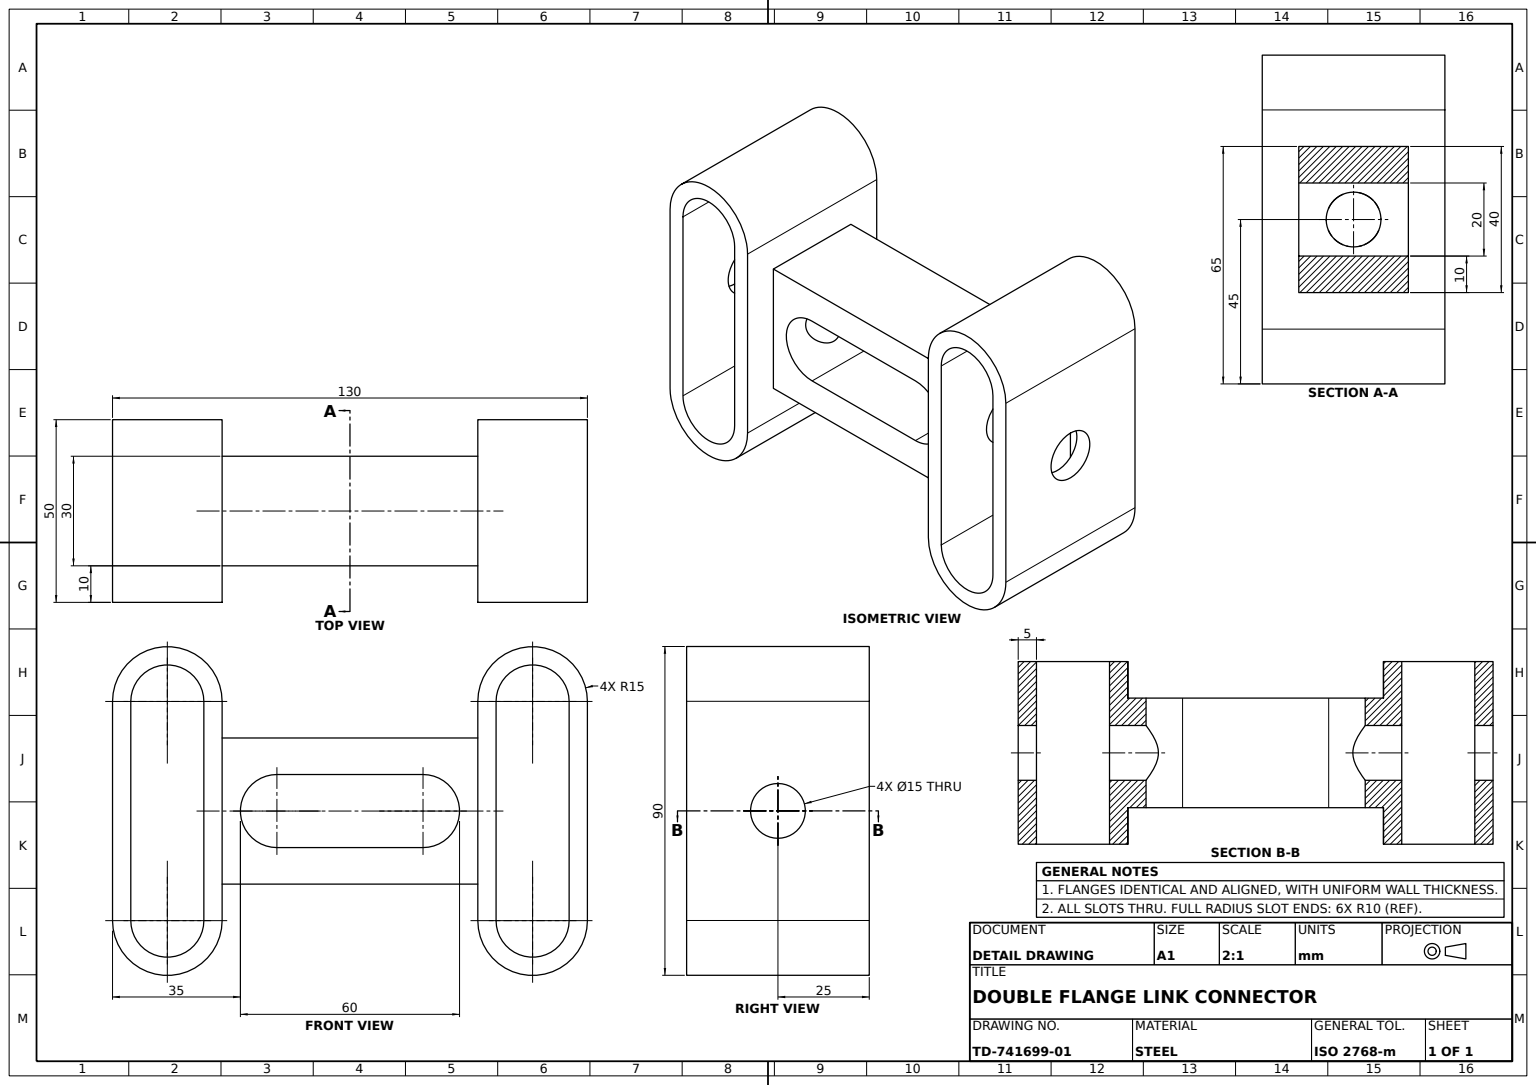
ISO-10303-21;
HEADER;
FILE_DESCRIPTION((''),'2;1');
FILE_NAME('','',(''),(''),'','','');
FILE_SCHEMA(('AUTOMOTIVE_DESIGN'));
ENDSEC;
DATA;
#1=APPLICATION_CONTEXT('');
#2=PRODUCT_CONTEXT('',#1,'mechanical');
#3=PRODUCT('','','',(#2));
#4=PRODUCT_DEFINITION_FORMATION('','',#3);
#5=PRODUCT_DEFINITION_CONTEXT('',#1,'design');
#6=PRODUCT_DEFINITION('','',#4,#5);
#7=PRODUCT_DEFINITION_SHAPE('','',#6);
#8=(LENGTH_UNIT()NAMED_UNIT(*)SI_UNIT(.MILLI.,.METRE.));
#9=(NAMED_UNIT(*)PLANE_ANGLE_UNIT()SI_UNIT($,.RADIAN.));
#10=(NAMED_UNIT(*)SI_UNIT($,.STERADIAN.)SOLID_ANGLE_UNIT());
#11=UNCERTAINTY_MEASURE_WITH_UNIT(LENGTH_MEASURE(0.005),#8,'distance_accuracy_value','');
#12=(GEOMETRIC_REPRESENTATION_CONTEXT(3)GLOBAL_UNCERTAINTY_ASSIGNED_CONTEXT((#11))GLOBAL_UNIT_ASSIGNED_CONTEXT((#8,#9,#10))REPRESENTATION_CONTEXT('',''));
#13=CARTESIAN_POINT('',(35.,15.,-20.));
#14=VERTEX_POINT('',#13);
#15=CARTESIAN_POINT('',(-35.,15.,-20.));
#16=VERTEX_POINT('',#15);
#17=CARTESIAN_POINT('',(65.,15.,-20.));
#18=DIRECTION('',(-1.,0.,0.));
#19=VECTOR('',#18,1000.);
#20=LINE('',#17,#19);
#21=EDGE_CURVE('',#14,#16,#20,.T.);
#22=ORIENTED_EDGE('',*,*,#21,.F.);
#23=CARTESIAN_POINT('',(35.,-15.,-20.));
#24=VERTEX_POINT('',#23);
#25=DIRECTION('',(0.,-1.,0.));
#26=VECTOR('',#25,1000.);
#27=LINE('',#23,#26);
#28=EDGE_CURVE('',#14,#24,#27,.T.);
#29=ORIENTED_EDGE('',*,*,#28,.T.);
#30=CARTESIAN_POINT('',(-35.,-15.,-20.));
#31=VERTEX_POINT('',#30);
#32=CARTESIAN_POINT('',(65.,-15.,-20.));
#33=LINE('',#32,#19);
#34=EDGE_CURVE('',#24,#31,#33,.T.);
#35=ORIENTED_EDGE('',*,*,#34,.T.);
#36=LINE('',#30,#26);
#37=EDGE_CURVE('',#16,#31,#36,.T.);
#38=ORIENTED_EDGE('',*,*,#37,.F.);
#39=EDGE_LOOP('',(#22,#29,#35,#38));
#40=FACE_BOUND('',#39,.T.);
#41=DIRECTION('',(0.,0.,-1.));
#42=AXIS2_PLACEMENT_3D('',#32,#41,#18);
#43=PLANE('',#42);
#44=ADVANCED_FACE('',(#40),#43,.T.);
#45=CARTESIAN_POINT('',(60.,25.,-30.));
#46=VERTEX_POINT('',#45);
#47=CARTESIAN_POINT('',(60.,-25.,-30.));
#48=VERTEX_POINT('',#47);
#49=CARTESIAN_POINT('',(60.,-51.,-30.));
#50=DIRECTION('',(0.,1.,0.));
#51=VECTOR('',#50,1000.);
#52=LINE('',#49,#51);
#53=EDGE_CURVE('',#46,#48,#52,.F.);
#54=ORIENTED_EDGE('',*,*,#53,.T.);
#55=CARTESIAN_POINT('',(60.,-25.,30.));
#56=VERTEX_POINT('',#55);
#57=VECTOR('',#41,1000.);
#58=LINE('',#55,#57);
#59=EDGE_CURVE('',#56,#48,#58,.T.);
#60=ORIENTED_EDGE('',*,*,#59,.F.);
#61=CARTESIAN_POINT('',(60.,25.,30.));
#62=VERTEX_POINT('',#61);
#63=CARTESIAN_POINT('',(60.,-51.,30.));
#64=LINE('',#63,#51);
#65=EDGE_CURVE('',#62,#56,#64,.F.);
#66=ORIENTED_EDGE('',*,*,#65,.F.);
#67=LINE('',#61,#57);
#68=EDGE_CURVE('',#62,#46,#67,.T.);
#69=ORIENTED_EDGE('',*,*,#68,.T.);
#70=EDGE_LOOP('',(#54,#60,#66,#69));
#71=FACE_BOUND('',#70,.T.);
#72=CARTESIAN_POINT('',(60.,0.,7.5));
#73=VERTEX_POINT('',#72);
#74=CARTESIAN_POINT('',(60.,0.,0.));
#75=DIRECTION('',(0.,0.,1.));
#76=AXIS2_PLACEMENT_3D('',#74,#18,#75);
#77=CIRCLE('',#76,7.5);
#78=EDGE_CURVE('',#73,#73,#77,.T.);
#79=ORIENTED_EDGE('',*,*,#78,.F.);
#80=EDGE_LOOP('',(#79));
#81=FACE_BOUND('',#80,.T.);
#82=AXIS2_PLACEMENT_3D('',#49,#18,#75);
#83=PLANE('',#82);
#84=ADVANCED_FACE('',(#71,#81),#83,.T.);
#85=CARTESIAN_POINT('',(40.,25.,-30.));
#86=VERTEX_POINT('',#85);
#87=CARTESIAN_POINT('',(50.,25.,-30.));
#88=AXIS2_PLACEMENT_3D('',#87,#25,#41);
#89=CIRCLE('',#88,10.);
#90=EDGE_CURVE('',#46,#86,#89,.F.);
#91=ORIENTED_EDGE('',*,*,#90,.T.);
#92=CARTESIAN_POINT('',(40.,-25.,-30.));
#93=VERTEX_POINT('',#92);
#94=CARTESIAN_POINT('',(40.,-51.,-30.));
#95=LINE('',#94,#51);
#96=EDGE_CURVE('',#86,#93,#95,.F.);
#97=ORIENTED_EDGE('',*,*,#96,.T.);
#98=CARTESIAN_POINT('',(50.,-25.,-30.));
#99=AXIS2_PLACEMENT_3D('',#98,#25,#41);
#100=CIRCLE('',#99,10.);
#101=EDGE_CURVE('',#48,#93,#100,.F.);
#102=ORIENTED_EDGE('',*,*,#101,.F.);
#103=ORIENTED_EDGE('',*,*,#53,.F.);
#104=EDGE_LOOP('',(#91,#97,#102,#103));
#105=FACE_BOUND('',#104,.T.);
#106=CARTESIAN_POINT('',(50.,-51.,-30.));
#107=AXIS2_PLACEMENT_3D('',#106,#50,#75);
#108=CYLINDRICAL_SURFACE('',#107,10.);
#109=ADVANCED_FACE('',(#105),#108,.F.);
#110=CARTESIAN_POINT('',(40.,0.,-7.5));
#111=VERTEX_POINT('',#110);
#112=CARTESIAN_POINT('',(40.,0.,0.));
#113=DIRECTION('',(1.,0.,0.));
#114=AXIS2_PLACEMENT_3D('',#112,#113,#41);
#115=CIRCLE('',#114,7.5);
#116=EDGE_CURVE('',#111,#111,#115,.T.);
#117=ORIENTED_EDGE('',*,*,#116,.T.);
#118=EDGE_LOOP('',(#117));
#119=FACE_BOUND('',#118,.T.);
#120=CARTESIAN_POINT('',(26.614378,0.,7.5));
#121=VERTEX_POINT('',#120);
#122=CARTESIAN_POINT('',(26.742202,-1.555656,7.390074));
#123=CARTESIAN_POINT('',(26.485198,0.527121,7.609599));
#124=CARTESIAN_POINT('',(27.137881,3.034196,7.063234));
#125=CARTESIAN_POINT('',(28.483267,5.377309,5.469181));
#126=CARTESIAN_POINT('',(29.650344,7.042163,3.112347));
#127=CARTESIAN_POINT('',(30.169282,7.721606,0.025455));
#128=CARTESIAN_POINT('',(29.672301,7.07111,-3.048672));
#129=CARTESIAN_POINT('',(28.494965,5.399488,-5.454098));
#130=CARTESIAN_POINT('',(27.380453,3.448516,-6.78143));
#131=CARTESIAN_POINT('',(26.74576,1.568514,-7.386559));
#132=CARTESIAN_POINT('',(26.551514,0.025291,-7.554237));
#133=CARTESIAN_POINT('',(26.734722,-1.523498,-7.396257));
#134=CARTESIAN_POINT('',(27.362431,-3.412182,-6.800946));
#135=CARTESIAN_POINT('',(28.477733,-5.372733,-5.475881));
#136=CARTESIAN_POINT('',(29.649907,-7.040721,-3.116164));
#137=CARTESIAN_POINT('',(30.169729,-7.722462,-0.025289));
#138=CARTESIAN_POINT('',(29.670957,-7.069137,3.05425));
#139=CARTESIAN_POINT('',(28.490958,-5.394144,5.460679));
#140=CARTESIAN_POINT('',(27.374214,-3.434962,6.787838));
#141=B_SPLINE_CURVE_WITH_KNOTS('',3,(#122,#123,#124,#125,#126,#127,#128,#129,#130,#131,#132,#133,#134,#135,#136,#137,#138,#139,#140,#122,#123,#124),.UNSPECIFIED.,.T.,.F.,(1,1,1,1,1,1,1,1,1,1,1,1,1,1,1,1,1,1,1,1,1,1,1,1,1,1),(-0.006118289,-0.003059145,-0.001529572,0.,0.003059145,0.006118289,0.009177434,0.012236578,0.015295723,0.018354867,0.021414012,0.022943584,0.024473156,0.026002728,0.027532301,0.030591445,0.03365059,0.036709734,0.039768879,0.042828023,0.045887168,0.04741674,0.048946312,0.052005457,0.055064601,0.058123746),.UNSPECIFIED.);
#142=EDGE_CURVE('',#121,#121,#141,.T.);
#143=ORIENTED_EDGE('',*,*,#142,.T.);
#144=EDGE_LOOP('',(#143));
#145=FACE_BOUND('',#144,.T.);
#146=CARTESIAN_POINT('',(65.,0.,0.));
#147=AXIS2_PLACEMENT_3D('',#146,#18,#75);
#148=CYLINDRICAL_SURFACE('',#147,7.5);
#149=ADVANCED_FACE('',(#119,#145),#148,.F.);
#150=ORIENTED_EDGE('',*,*,#78,.T.);
#151=EDGE_LOOP('',(#150));
#152=FACE_BOUND('',#151,.T.);
#153=CARTESIAN_POINT('',(65.,0.,7.5));
#154=VERTEX_POINT('',#153);
#155=CIRCLE('',#147,7.5);
#156=EDGE_CURVE('',#154,#154,#155,.T.);
#157=ORIENTED_EDGE('',*,*,#156,.F.);
#158=EDGE_LOOP('',(#157));
#159=FACE_BOUND('',#158,.T.);
#160=ADVANCED_FACE('',(#152,#159),#148,.F.);
#161=CARTESIAN_POINT('',(20.,15.,10.));
#162=VERTEX_POINT('',#161);
#163=CARTESIAN_POINT('',(20.,-15.,10.));
#164=VERTEX_POINT('',#163);
#165=CARTESIAN_POINT('',(20.,-51.,10.));
#166=LINE('',#165,#51);
#167=EDGE_CURVE('',#162,#164,#166,.F.);
#168=ORIENTED_EDGE('',*,*,#167,.T.);
#169=CARTESIAN_POINT('',(-20.,-15.,10.));
#170=VERTEX_POINT('',#169);
#171=CARTESIAN_POINT('',(0.,-15.,10.));
#172=LINE('',#171,#19);
#173=EDGE_CURVE('',#164,#170,#172,.T.);
#174=ORIENTED_EDGE('',*,*,#173,.T.);
#175=CARTESIAN_POINT('',(-20.,15.,10.));
#176=VERTEX_POINT('',#175);
#177=CARTESIAN_POINT('',(-20.,-51.,10.));
#178=LINE('',#177,#51);
#179=EDGE_CURVE('',#176,#170,#178,.F.);
#180=ORIENTED_EDGE('',*,*,#179,.F.);
#181=CARTESIAN_POINT('',(0.,15.,10.));
#182=LINE('',#181,#19);
#183=EDGE_CURVE('',#162,#176,#182,.T.);
#184=ORIENTED_EDGE('',*,*,#183,.F.);
#185=EDGE_LOOP('',(#168,#174,#180,#184));
#186=FACE_BOUND('',#185,.T.);
#187=AXIS2_PLACEMENT_3D('',#165,#41,#18);
#188=PLANE('',#187);
#189=ADVANCED_FACE('',(#186),#188,.T.);
#190=CARTESIAN_POINT('',(65.,25.,30.));
#191=VERTEX_POINT('',#190);
#192=CARTESIAN_POINT('',(35.,25.,30.));
#193=VERTEX_POINT('',#192);
#194=CARTESIAN_POINT('',(50.,25.,30.));
#195=AXIS2_PLACEMENT_3D('',#194,#25,#113);
#196=CIRCLE('',#195,15.);
#197=EDGE_CURVE('',#191,#193,#196,.T.);
#198=ORIENTED_EDGE('',*,*,#197,.F.);
#199=CARTESIAN_POINT('',(65.,25.,-30.));
#200=VERTEX_POINT('',#199);
#201=VECTOR('',#75,1000.);
#202=LINE('',#199,#201);
#203=EDGE_CURVE('',#200,#191,#202,.T.);
#204=ORIENTED_EDGE('',*,*,#203,.F.);
#205=CARTESIAN_POINT('',(35.,25.,-30.));
#206=VERTEX_POINT('',#205);
#207=AXIS2_PLACEMENT_3D('',#87,#25,#113);
#208=CIRCLE('',#207,15.);
#209=EDGE_CURVE('',#206,#200,#208,.T.);
#210=ORIENTED_EDGE('',*,*,#209,.F.);
#211=LINE('',#192,#57);
#212=EDGE_CURVE('',#193,#206,#211,.T.);
#213=ORIENTED_EDGE('',*,*,#212,.F.);
#214=EDGE_LOOP('',(#198,#204,#210,#213));
#215=FACE_BOUND('',#214,.T.);
#216=CARTESIAN_POINT('',(40.,25.,30.));
#217=VERTEX_POINT('',#216);
#218=AXIS2_PLACEMENT_3D('',#194,#25,#41);
#219=CIRCLE('',#218,10.);
#220=EDGE_CURVE('',#217,#62,#219,.F.);
#221=ORIENTED_EDGE('',*,*,#220,.F.);
#222=LINE('',#216,#201);
#223=EDGE_CURVE('',#86,#217,#222,.T.);
#224=ORIENTED_EDGE('',*,*,#223,.F.);
#225=ORIENTED_EDGE('',*,*,#90,.F.);
#226=ORIENTED_EDGE('',*,*,#68,.F.);
#227=EDGE_LOOP('',(#221,#224,#225,#226));
#228=FACE_BOUND('',#227,.T.);
#229=PLANE('',#218);
#230=ADVANCED_FACE('',(#215,#228),#229,.F.);
#231=CARTESIAN_POINT('',(-60.,0.,7.5));
#232=VERTEX_POINT('',#231);
#233=CARTESIAN_POINT('',(-60.,0.,0.));
#234=AXIS2_PLACEMENT_3D('',#233,#18,#75);
#235=CIRCLE('',#234,7.5);
#236=EDGE_CURVE('',#232,#232,#235,.T.);
#237=ORIENTED_EDGE('',*,*,#236,.T.);
#238=EDGE_LOOP('',(#237));
#239=FACE_BOUND('',#238,.T.);
#240=CARTESIAN_POINT('',(-60.,-25.,-30.));
#241=VERTEX_POINT('',#240);
#242=CARTESIAN_POINT('',(-60.,-25.,30.));
#243=VERTEX_POINT('',#242);
#244=LINE('',#242,#201);
#245=EDGE_CURVE('',#241,#243,#244,.T.);
#246=ORIENTED_EDGE('',*,*,#245,.F.);
#247=CARTESIAN_POINT('',(-60.,25.,-30.));
#248=VERTEX_POINT('',#247);
#249=CARTESIAN_POINT('',(-60.,-51.,-30.));
#250=LINE('',#249,#51);
#251=EDGE_CURVE('',#248,#241,#250,.F.);
#252=ORIENTED_EDGE('',*,*,#251,.F.);
#253=CARTESIAN_POINT('',(-60.,25.,30.));
#254=VERTEX_POINT('',#253);
#255=LINE('',#253,#201);
#256=EDGE_CURVE('',#248,#254,#255,.T.);
#257=ORIENTED_EDGE('',*,*,#256,.T.);
#258=CARTESIAN_POINT('',(-60.,-51.,30.));
#259=LINE('',#258,#51);
#260=EDGE_CURVE('',#254,#243,#259,.F.);
#261=ORIENTED_EDGE('',*,*,#260,.T.);
#262=EDGE_LOOP('',(#246,#252,#257,#261));
#263=FACE_BOUND('',#262,.T.);
#264=AXIS2_PLACEMENT_3D('',#249,#18,#75);
#265=PLANE('',#264);
#266=ADVANCED_FACE('',(#239,#263),#265,.F.);
#267=ORIENTED_EDGE('',*,*,#220,.T.);
#268=ORIENTED_EDGE('',*,*,#65,.T.);
#269=CARTESIAN_POINT('',(40.,-25.,30.));
#270=VERTEX_POINT('',#269);
#271=CARTESIAN_POINT('',(50.,-25.,30.));
#272=AXIS2_PLACEMENT_3D('',#271,#25,#41);
#273=CIRCLE('',#272,10.);
#274=EDGE_CURVE('',#270,#56,#273,.F.);
#275=ORIENTED_EDGE('',*,*,#274,.F.);
#276=CARTESIAN_POINT('',(40.,-51.,30.));
#277=LINE('',#276,#51);
#278=EDGE_CURVE('',#217,#270,#277,.F.);
#279=ORIENTED_EDGE('',*,*,#278,.F.);
#280=EDGE_LOOP('',(#267,#268,#275,#279));
#281=FACE_BOUND('',#280,.T.);
#282=CARTESIAN_POINT('',(50.,-51.,30.));
#283=AXIS2_PLACEMENT_3D('',#282,#50,#75);
#284=CYLINDRICAL_SURFACE('',#283,10.);
#285=ADVANCED_FACE('',(#281),#284,.F.);
#286=ORIENTED_EDGE('',*,*,#116,.F.);
#287=EDGE_LOOP('',(#286));
#288=FACE_BOUND('',#287,.T.);
#289=ORIENTED_EDGE('',*,*,#278,.T.);
#290=LINE('',#269,#201);
#291=EDGE_CURVE('',#93,#270,#290,.T.);
#292=ORIENTED_EDGE('',*,*,#291,.F.);
#293=ORIENTED_EDGE('',*,*,#96,.F.);
#294=ORIENTED_EDGE('',*,*,#223,.T.);
#295=EDGE_LOOP('',(#289,#292,#293,#294));
#296=FACE_BOUND('',#295,.T.);
#297=AXIS2_PLACEMENT_3D('',#276,#113,#41);
#298=PLANE('',#297);
#299=ADVANCED_FACE('',(#288,#296),#298,.T.);
#300=CARTESIAN_POINT('',(35.,-25.,-30.));
#301=VERTEX_POINT('',#300);
#302=LINE('',#300,#51);
#303=EDGE_CURVE('',#301,#206,#302,.T.);
#304=ORIENTED_EDGE('',*,*,#303,.T.);
#305=ORIENTED_EDGE('',*,*,#209,.T.);
#306=CARTESIAN_POINT('',(65.,-25.,-30.));
#307=VERTEX_POINT('',#306);
#308=LINE('',#306,#51);
#309=EDGE_CURVE('',#307,#200,#308,.T.);
#310=ORIENTED_EDGE('',*,*,#309,.F.);
#311=AXIS2_PLACEMENT_3D('',#98,#25,#113);
#312=CIRCLE('',#311,15.);
#313=EDGE_CURVE('',#301,#307,#312,.T.);
#314=ORIENTED_EDGE('',*,*,#313,.F.);
#315=EDGE_LOOP('',(#304,#305,#310,#314));
#316=FACE_BOUND('',#315,.T.);
#317=AXIS2_PLACEMENT_3D('',#98,#50,#75);
#318=CYLINDRICAL_SURFACE('',#317,15.);
#319=ADVANCED_FACE('',(#316),#318,.T.);
#320=CARTESIAN_POINT('',(-40.,0.,-7.5));
#321=VERTEX_POINT('',#320);
#322=CARTESIAN_POINT('',(-40.,0.,0.));
#323=AXIS2_PLACEMENT_3D('',#322,#113,#41);
#324=CIRCLE('',#323,7.5);
#325=EDGE_CURVE('',#321,#321,#324,.T.);
#326=ORIENTED_EDGE('',*,*,#325,.T.);
#327=EDGE_LOOP('',(#326));
#328=FACE_BOUND('',#327,.T.);
#329=CARTESIAN_POINT('',(-40.,-25.,30.));
#330=VERTEX_POINT('',#329);
#331=CARTESIAN_POINT('',(-40.,-25.,-30.));
#332=VERTEX_POINT('',#331);
#333=LINE('',#329,#57);
#334=EDGE_CURVE('',#330,#332,#333,.T.);
#335=ORIENTED_EDGE('',*,*,#334,.F.);
#336=CARTESIAN_POINT('',(-40.,25.,30.));
#337=VERTEX_POINT('',#336);
#338=CARTESIAN_POINT('',(-40.,-51.,30.));
#339=LINE('',#338,#51);
#340=EDGE_CURVE('',#337,#330,#339,.F.);
#341=ORIENTED_EDGE('',*,*,#340,.F.);
#342=CARTESIAN_POINT('',(-40.,25.,-30.));
#343=VERTEX_POINT('',#342);
#344=LINE('',#336,#57);
#345=EDGE_CURVE('',#337,#343,#344,.T.);
#346=ORIENTED_EDGE('',*,*,#345,.T.);
#347=CARTESIAN_POINT('',(-40.,-51.,-30.));
#348=LINE('',#347,#51);
#349=EDGE_CURVE('',#343,#332,#348,.F.);
#350=ORIENTED_EDGE('',*,*,#349,.T.);
#351=EDGE_LOOP('',(#335,#341,#346,#350));
#352=FACE_BOUND('',#351,.T.);
#353=AXIS2_PLACEMENT_3D('',#338,#113,#41);
#354=PLANE('',#353);
#355=ADVANCED_FACE('',(#328,#352),#354,.F.);
#356=CARTESIAN_POINT('',(-50.,-25.,-30.));
#357=AXIS2_PLACEMENT_3D('',#356,#50,#75);
#358=CIRCLE('',#357,10.);
#359=EDGE_CURVE('',#332,#241,#358,.T.);
#360=ORIENTED_EDGE('',*,*,#359,.T.);
#361=ORIENTED_EDGE('',*,*,#245,.T.);
#362=CARTESIAN_POINT('',(-50.,-25.,30.));
#363=AXIS2_PLACEMENT_3D('',#362,#50,#75);
#364=CIRCLE('',#363,10.);
#365=EDGE_CURVE('',#243,#330,#364,.T.);
#366=ORIENTED_EDGE('',*,*,#365,.T.);
#367=ORIENTED_EDGE('',*,*,#334,.T.);
#368=EDGE_LOOP('',(#360,#361,#366,#367));
#369=FACE_BOUND('',#368,.T.);
#370=CARTESIAN_POINT('',(-65.,-25.,-30.));
#371=VERTEX_POINT('',#370);
#372=CARTESIAN_POINT('',(-65.,-25.,30.));
#373=VERTEX_POINT('',#372);
#374=LINE('',#370,#201);
#375=EDGE_CURVE('',#371,#373,#374,.T.);
#376=ORIENTED_EDGE('',*,*,#375,.F.);
#377=CARTESIAN_POINT('',(-35.,-25.,-30.));
#378=VERTEX_POINT('',#377);
#379=AXIS2_PLACEMENT_3D('',#356,#50,#18);
#380=CIRCLE('',#379,15.);
#381=EDGE_CURVE('',#378,#371,#380,.T.);
#382=ORIENTED_EDGE('',*,*,#381,.F.);
#383=CARTESIAN_POINT('',(-35.,-25.,30.));
#384=VERTEX_POINT('',#383);
#385=LINE('',#383,#57);
#386=EDGE_CURVE('',#384,#378,#385,.T.);
#387=ORIENTED_EDGE('',*,*,#386,.F.);
#388=AXIS2_PLACEMENT_3D('',#362,#50,#18);
#389=CIRCLE('',#388,15.);
#390=EDGE_CURVE('',#373,#384,#389,.T.);
#391=ORIENTED_EDGE('',*,*,#390,.F.);
#392=EDGE_LOOP('',(#376,#382,#387,#391));
#393=FACE_BOUND('',#392,.T.);
#394=PLANE('',#363);
#395=ADVANCED_FACE('',(#369,#393),#394,.F.);
#396=CARTESIAN_POINT('',(20.,15.,-10.));
#397=VERTEX_POINT('',#396);
#398=CARTESIAN_POINT('',(20.,15.,0.));
#399=AXIS2_PLACEMENT_3D('',#398,#50,#75);
#400=CIRCLE('',#399,10.);
#401=EDGE_CURVE('',#397,#162,#400,.F.);
#402=ORIENTED_EDGE('',*,*,#401,.F.);
#403=CARTESIAN_POINT('',(20.,-15.,-10.));
#404=VERTEX_POINT('',#403);
#405=CARTESIAN_POINT('',(20.,-51.,-10.));
#406=LINE('',#405,#51);
#407=EDGE_CURVE('',#397,#404,#406,.F.);
#408=ORIENTED_EDGE('',*,*,#407,.T.);
#409=CARTESIAN_POINT('',(20.,-15.,0.));
#410=AXIS2_PLACEMENT_3D('',#409,#50,#75);
#411=CIRCLE('',#410,10.);
#412=EDGE_CURVE('',#404,#164,#411,.F.);
#413=ORIENTED_EDGE('',*,*,#412,.T.);
#414=ORIENTED_EDGE('',*,*,#167,.F.);
#415=EDGE_LOOP('',(#402,#408,#413,#414));
#416=FACE_BOUND('',#415,.T.);
#417=ORIENTED_EDGE('',*,*,#142,.F.);
#418=EDGE_LOOP('',(#417));
#419=FACE_BOUND('',#418,.T.);
#420=CARTESIAN_POINT('',(20.,-51.,0.));
#421=AXIS2_PLACEMENT_3D('',#420,#50,#75);
#422=CYLINDRICAL_SURFACE('',#421,10.);
#423=ADVANCED_FACE('',(#416,#419),#422,.F.);
#424=CARTESIAN_POINT('',(-50.,25.,30.));
#425=AXIS2_PLACEMENT_3D('',#424,#50,#75);
#426=CIRCLE('',#425,10.);
#427=EDGE_CURVE('',#254,#337,#426,.T.);
#428=ORIENTED_EDGE('',*,*,#427,.F.);
#429=ORIENTED_EDGE('',*,*,#256,.F.);
#430=CARTESIAN_POINT('',(-50.,25.,-30.));
#431=AXIS2_PLACEMENT_3D('',#430,#50,#75);
#432=CIRCLE('',#431,10.);
#433=EDGE_CURVE('',#343,#248,#432,.T.);
#434=ORIENTED_EDGE('',*,*,#433,.F.);
#435=ORIENTED_EDGE('',*,*,#345,.F.);
#436=EDGE_LOOP('',(#428,#429,#434,#435));
#437=FACE_BOUND('',#436,.T.);
#438=CARTESIAN_POINT('',(-35.,25.,-30.));
#439=VERTEX_POINT('',#438);
#440=CARTESIAN_POINT('',(-65.,25.,-30.));
#441=VERTEX_POINT('',#440);
#442=AXIS2_PLACEMENT_3D('',#430,#50,#18);
#443=CIRCLE('',#442,15.);
#444=EDGE_CURVE('',#439,#441,#443,.T.);
#445=ORIENTED_EDGE('',*,*,#444,.T.);
#446=CARTESIAN_POINT('',(-65.,25.,30.));
#447=VERTEX_POINT('',#446);
#448=LINE('',#440,#201);
#449=EDGE_CURVE('',#441,#447,#448,.T.);
#450=ORIENTED_EDGE('',*,*,#449,.T.);
#451=CARTESIAN_POINT('',(-35.,25.,30.));
#452=VERTEX_POINT('',#451);
#453=AXIS2_PLACEMENT_3D('',#424,#50,#18);
#454=CIRCLE('',#453,15.);
#455=EDGE_CURVE('',#447,#452,#454,.T.);
#456=ORIENTED_EDGE('',*,*,#455,.T.);
#457=LINE('',#451,#57);
#458=EDGE_CURVE('',#452,#439,#457,.T.);
#459=ORIENTED_EDGE('',*,*,#458,.T.);
#460=EDGE_LOOP('',(#445,#450,#456,#459));
#461=FACE_BOUND('',#460,.T.);
#462=PLANE('',#425);
#463=ADVANCED_FACE('',(#437,#461),#462,.T.);
#464=CARTESIAN_POINT('',(-20.,15.,-10.));
#465=VERTEX_POINT('',#464);
#466=CARTESIAN_POINT('',(-20.,15.,0.));
#467=AXIS2_PLACEMENT_3D('',#466,#50,#75);
#468=CIRCLE('',#467,10.);
#469=EDGE_CURVE('',#176,#465,#468,.F.);
#470=ORIENTED_EDGE('',*,*,#469,.F.);
#471=ORIENTED_EDGE('',*,*,#179,.T.);
#472=CARTESIAN_POINT('',(-20.,-15.,-10.));
#473=VERTEX_POINT('',#472);
#474=CARTESIAN_POINT('',(-20.,-15.,0.));
#475=AXIS2_PLACEMENT_3D('',#474,#50,#75);
#476=CIRCLE('',#475,10.);
#477=EDGE_CURVE('',#170,#473,#476,.F.);
#478=ORIENTED_EDGE('',*,*,#477,.T.);
#479=CARTESIAN_POINT('',(-20.,-51.,-10.));
#480=LINE('',#479,#51);
#481=EDGE_CURVE('',#465,#473,#480,.F.);
#482=ORIENTED_EDGE('',*,*,#481,.F.);
#483=EDGE_LOOP('',(#470,#471,#478,#482));
#484=FACE_BOUND('',#483,.T.);
#485=CARTESIAN_POINT('',(-26.614378,0.,7.5));
#486=VERTEX_POINT('',#485);
#487=CARTESIAN_POINT('',(-26.742202,1.555656,7.390074));
#488=CARTESIAN_POINT('',(-26.485198,-0.527121,7.609599));
#489=CARTESIAN_POINT('',(-27.137881,-3.034196,7.063234));
#490=CARTESIAN_POINT('',(-28.483267,-5.377309,5.469181));
#491=CARTESIAN_POINT('',(-29.650344,-7.042163,3.112347));
#492=CARTESIAN_POINT('',(-30.169282,-7.721606,0.025455));
#493=CARTESIAN_POINT('',(-29.672301,-7.07111,-3.048672));
#494=CARTESIAN_POINT('',(-28.494965,-5.399488,-5.454098));
#495=CARTESIAN_POINT('',(-27.380453,-3.448516,-6.78143));
#496=CARTESIAN_POINT('',(-26.74576,-1.568514,-7.386559));
#497=CARTESIAN_POINT('',(-26.551514,-0.025291,-7.554237));
#498=CARTESIAN_POINT('',(-26.734722,1.523498,-7.396257));
#499=CARTESIAN_POINT('',(-27.362431,3.412182,-6.800946));
#500=CARTESIAN_POINT('',(-28.477733,5.372733,-5.475881));
#501=CARTESIAN_POINT('',(-29.649907,7.040721,-3.116164));
#502=CARTESIAN_POINT('',(-30.169729,7.722462,-0.025289));
#503=CARTESIAN_POINT('',(-29.670957,7.069137,3.05425));
#504=CARTESIAN_POINT('',(-28.490958,5.394144,5.460679));
#505=CARTESIAN_POINT('',(-27.374214,3.434962,6.787838));
#506=B_SPLINE_CURVE_WITH_KNOTS('',3,(#487,#488,#489,#490,#491,#492,#493,#494,#495,#496,#497,#498,#499,#500,#501,#502,#503,#504,#505,#487,#488,#489),.UNSPECIFIED.,.T.,.F.,(1,1,1,1,1,1,1,1,1,1,1,1,1,1,1,1,1,1,1,1,1,1,1,1,1,1),(-0.006118289,-0.003059145,-0.001529572,0.,0.003059145,0.006118289,0.009177434,0.012236578,0.015295723,0.018354867,0.021414012,0.022943584,0.024473156,0.026002728,0.027532301,0.030591445,0.03365059,0.036709734,0.039768879,0.042828023,0.045887168,0.04741674,0.048946312,0.052005457,0.055064601,0.058123746),.UNSPECIFIED.);
#507=EDGE_CURVE('',#486,#486,#506,.T.);
#508=ORIENTED_EDGE('',*,*,#507,.F.);
#509=EDGE_LOOP('',(#508));
#510=FACE_BOUND('',#509,.T.);
#511=CARTESIAN_POINT('',(-20.,-51.,0.));
#512=AXIS2_PLACEMENT_3D('',#511,#50,#75);
#513=CYLINDRICAL_SURFACE('',#512,10.);
#514=ADVANCED_FACE('',(#484,#510),#513,.F.);
#515=CARTESIAN_POINT('',(0.,15.,-10.));
#516=VECTOR('',#113,1000.);
#517=LINE('',#515,#516);
#518=EDGE_CURVE('',#465,#397,#517,.T.);
#519=ORIENTED_EDGE('',*,*,#518,.T.);
#520=ORIENTED_EDGE('',*,*,#401,.T.);
#521=ORIENTED_EDGE('',*,*,#183,.T.);
#522=ORIENTED_EDGE('',*,*,#469,.T.);
#523=EDGE_LOOP('',(#519,#520,#521,#522));
#524=FACE_BOUND('',#523,.T.);
#525=CARTESIAN_POINT('',(35.,15.,20.));
#526=VERTEX_POINT('',#525);
#527=CARTESIAN_POINT('',(35.,15.,0.));
#528=LINE('',#527,#57);
#529=EDGE_CURVE('',#14,#526,#528,.F.);
#530=ORIENTED_EDGE('',*,*,#529,.F.);
#531=ORIENTED_EDGE('',*,*,#21,.T.);
#532=CARTESIAN_POINT('',(-35.,15.,20.));
#533=VERTEX_POINT('',#532);
#534=CARTESIAN_POINT('',(-35.,15.,0.));
#535=LINE('',#534,#57);
#536=EDGE_CURVE('',#16,#533,#535,.F.);
#537=ORIENTED_EDGE('',*,*,#536,.T.);
#538=CARTESIAN_POINT('',(-65.,15.,20.));
#539=LINE('',#538,#516);
#540=EDGE_CURVE('',#533,#526,#539,.T.);
#541=ORIENTED_EDGE('',*,*,#540,.T.);
#542=EDGE_LOOP('',(#530,#531,#537,#541));
#543=FACE_BOUND('',#542,.T.);
#544=CARTESIAN_POINT('',(0.,15.,0.));
#545=AXIS2_PLACEMENT_3D('',#544,#50,#75);
#546=PLANE('',#545);
#547=ADVANCED_FACE('',(#524,#543),#546,.T.);
#548=ORIENTED_EDGE('',*,*,#325,.F.);
#549=EDGE_LOOP('',(#548));
#550=FACE_BOUND('',#549,.T.);
#551=ORIENTED_EDGE('',*,*,#507,.T.);
#552=EDGE_LOOP('',(#551));
#553=FACE_BOUND('',#552,.T.);
#554=ADVANCED_FACE('',(#550,#553),#148,.F.);
#555=CARTESIAN_POINT('',(35.,-15.,20.));
#556=VERTEX_POINT('',#555);
#557=LINE('',#555,#51);
#558=EDGE_CURVE('',#556,#526,#557,.T.);
#559=ORIENTED_EDGE('',*,*,#558,.F.);
#560=CARTESIAN_POINT('',(35.,-15.,0.));
#561=LINE('',#560,#57);
#562=EDGE_CURVE('',#24,#556,#561,.F.);
#563=ORIENTED_EDGE('',*,*,#562,.F.);
#564=ORIENTED_EDGE('',*,*,#28,.F.);
#565=ORIENTED_EDGE('',*,*,#529,.T.);
#566=EDGE_LOOP('',(#559,#563,#564,#565));
#567=FACE_BOUND('',#566,.T.);
#568=ORIENTED_EDGE('',*,*,#212,.T.);
#569=ORIENTED_EDGE('',*,*,#303,.F.);
#570=CARTESIAN_POINT('',(35.,-25.,30.));
#571=VERTEX_POINT('',#570);
#572=LINE('',#570,#57);
#573=EDGE_CURVE('',#571,#301,#572,.T.);
#574=ORIENTED_EDGE('',*,*,#573,.F.);
#575=LINE('',#570,#51);
#576=EDGE_CURVE('',#571,#193,#575,.T.);
#577=ORIENTED_EDGE('',*,*,#576,.T.);
#578=EDGE_LOOP('',(#568,#569,#574,#577));
#579=FACE_BOUND('',#578,.T.);
#580=AXIS2_PLACEMENT_3D('',#570,#113,#41);
#581=PLANE('',#580);
#582=ADVANCED_FACE('',(#567,#579),#581,.F.);
#583=ORIENTED_EDGE('',*,*,#260,.F.);
#584=ORIENTED_EDGE('',*,*,#427,.T.);
#585=ORIENTED_EDGE('',*,*,#340,.T.);
#586=ORIENTED_EDGE('',*,*,#365,.F.);
#587=EDGE_LOOP('',(#583,#584,#585,#586));
#588=FACE_BOUND('',#587,.T.);
#589=CARTESIAN_POINT('',(-50.,-51.,30.));
#590=AXIS2_PLACEMENT_3D('',#589,#50,#75);
#591=CYLINDRICAL_SURFACE('',#590,10.);
#592=ADVANCED_FACE('',(#588),#591,.F.);
#593=CARTESIAN_POINT('',(-65.,0.,7.5));
#594=VERTEX_POINT('',#593);
#595=CARTESIAN_POINT('',(-65.,0.,0.));
#596=AXIS2_PLACEMENT_3D('',#595,#18,#75);
#597=CIRCLE('',#596,7.5);
#598=EDGE_CURVE('',#594,#594,#597,.T.);
#599=ORIENTED_EDGE('',*,*,#598,.T.);
#600=EDGE_LOOP('',(#599));
#601=FACE_BOUND('',#600,.T.);
#602=ORIENTED_EDGE('',*,*,#236,.F.);
#603=EDGE_LOOP('',(#602));
#604=FACE_BOUND('',#603,.T.);
#605=ADVANCED_FACE('',(#601,#604),#148,.F.);
#606=ORIENTED_EDGE('',*,*,#173,.F.);
#607=ORIENTED_EDGE('',*,*,#412,.F.);
#608=CARTESIAN_POINT('',(0.,-15.,-10.));
#609=LINE('',#608,#516);
#610=EDGE_CURVE('',#473,#404,#609,.T.);
#611=ORIENTED_EDGE('',*,*,#610,.F.);
#612=ORIENTED_EDGE('',*,*,#477,.F.);
#613=EDGE_LOOP('',(#606,#607,#611,#612));
#614=FACE_BOUND('',#613,.T.);
#615=CARTESIAN_POINT('',(-35.,-15.,20.));
#616=VERTEX_POINT('',#615);
#617=CARTESIAN_POINT('',(-35.,-15.,0.));
#618=LINE('',#617,#57);
#619=EDGE_CURVE('',#31,#616,#618,.F.);
#620=ORIENTED_EDGE('',*,*,#619,.F.);
#621=ORIENTED_EDGE('',*,*,#34,.F.);
#622=ORIENTED_EDGE('',*,*,#562,.T.);
#623=CARTESIAN_POINT('',(-65.,-15.,20.));
#624=LINE('',#623,#516);
#625=EDGE_CURVE('',#616,#556,#624,.T.);
#626=ORIENTED_EDGE('',*,*,#625,.F.);
#627=EDGE_LOOP('',(#620,#621,#622,#626));
#628=FACE_BOUND('',#627,.T.);
#629=CARTESIAN_POINT('',(0.,-15.,0.));
#630=AXIS2_PLACEMENT_3D('',#629,#50,#75);
#631=PLANE('',#630);
#632=ADVANCED_FACE('',(#614,#628),#631,.F.);
#633=LINE('',#615,#51);
#634=EDGE_CURVE('',#616,#533,#633,.T.);
#635=ORIENTED_EDGE('',*,*,#634,.T.);
#636=ORIENTED_EDGE('',*,*,#536,.F.);
#637=ORIENTED_EDGE('',*,*,#37,.T.);
#638=ORIENTED_EDGE('',*,*,#619,.T.);
#639=EDGE_LOOP('',(#635,#636,#637,#638));
#640=FACE_BOUND('',#639,.T.);
#641=LINE('',#383,#51);
#642=EDGE_CURVE('',#384,#452,#641,.T.);
#643=ORIENTED_EDGE('',*,*,#642,.F.);
#644=ORIENTED_EDGE('',*,*,#386,.T.);
#645=LINE('',#377,#51);
#646=EDGE_CURVE('',#378,#439,#645,.T.);
#647=ORIENTED_EDGE('',*,*,#646,.T.);
#648=ORIENTED_EDGE('',*,*,#458,.F.);
#649=EDGE_LOOP('',(#643,#644,#647,#648));
#650=FACE_BOUND('',#649,.T.);
#651=AXIS2_PLACEMENT_3D('',#383,#113,#41);
#652=PLANE('',#651);
#653=ADVANCED_FACE('',(#640,#650),#652,.T.);
#654=CARTESIAN_POINT('',(65.,-25.,30.));
#655=VERTEX_POINT('',#654);
#656=AXIS2_PLACEMENT_3D('',#271,#25,#113);
#657=CIRCLE('',#656,15.);
#658=EDGE_CURVE('',#655,#571,#657,.T.);
#659=ORIENTED_EDGE('',*,*,#658,.T.);
#660=ORIENTED_EDGE('',*,*,#573,.T.);
#661=ORIENTED_EDGE('',*,*,#313,.T.);
#662=LINE('',#306,#201);
#663=EDGE_CURVE('',#307,#655,#662,.T.);
#664=ORIENTED_EDGE('',*,*,#663,.T.);
#665=EDGE_LOOP('',(#659,#660,#661,#664));
#666=FACE_BOUND('',#665,.T.);
#667=ORIENTED_EDGE('',*,*,#291,.T.);
#668=ORIENTED_EDGE('',*,*,#274,.T.);
#669=ORIENTED_EDGE('',*,*,#59,.T.);
#670=ORIENTED_EDGE('',*,*,#101,.T.);
#671=EDGE_LOOP('',(#667,#668,#669,#670));
#672=FACE_BOUND('',#671,.T.);
#673=PLANE('',#272);
#674=ADVANCED_FACE('',(#666,#672),#673,.T.);
#675=ORIENTED_EDGE('',*,*,#598,.F.);
#676=EDGE_LOOP('',(#675));
#677=FACE_BOUND('',#676,.T.);
#678=LINE('',#372,#51);
#679=EDGE_CURVE('',#373,#447,#678,.T.);
#680=ORIENTED_EDGE('',*,*,#679,.T.);
#681=ORIENTED_EDGE('',*,*,#449,.F.);
#682=LINE('',#370,#51);
#683=EDGE_CURVE('',#371,#441,#682,.T.);
#684=ORIENTED_EDGE('',*,*,#683,.F.);
#685=ORIENTED_EDGE('',*,*,#375,.T.);
#686=EDGE_LOOP('',(#680,#681,#684,#685));
#687=FACE_BOUND('',#686,.T.);
#688=CARTESIAN_POINT('',(-65.,-15.,-20.));
#689=AXIS2_PLACEMENT_3D('',#688,#18,#75);
#690=PLANE('',#689);
#691=ADVANCED_FACE('',(#677,#687),#690,.T.);
#692=LINE('',#654,#51);
#693=EDGE_CURVE('',#655,#191,#692,.T.);
#694=ORIENTED_EDGE('',*,*,#693,.T.);
#695=ORIENTED_EDGE('',*,*,#197,.T.);
#696=ORIENTED_EDGE('',*,*,#576,.F.);
#697=ORIENTED_EDGE('',*,*,#658,.F.);
#698=EDGE_LOOP('',(#694,#695,#696,#697));
#699=FACE_BOUND('',#698,.T.);
#700=AXIS2_PLACEMENT_3D('',#271,#50,#75);
#701=CYLINDRICAL_SURFACE('',#700,15.);
#702=ADVANCED_FACE('',(#699),#701,.T.);
#703=ORIENTED_EDGE('',*,*,#683,.T.);
#704=ORIENTED_EDGE('',*,*,#444,.F.);
#705=ORIENTED_EDGE('',*,*,#646,.F.);
#706=ORIENTED_EDGE('',*,*,#381,.T.);
#707=EDGE_LOOP('',(#703,#704,#705,#706));
#708=FACE_BOUND('',#707,.T.);
#709=CYLINDRICAL_SURFACE('',#357,15.);
#710=ADVANCED_FACE('',(#708),#709,.T.);
#711=ORIENTED_EDGE('',*,*,#634,.F.);
#712=ORIENTED_EDGE('',*,*,#625,.T.);
#713=ORIENTED_EDGE('',*,*,#558,.T.);
#714=ORIENTED_EDGE('',*,*,#540,.F.);
#715=EDGE_LOOP('',(#711,#712,#713,#714));
#716=FACE_BOUND('',#715,.T.);
#717=AXIS2_PLACEMENT_3D('',#623,#75,#113);
#718=PLANE('',#717);
#719=ADVANCED_FACE('',(#716),#718,.T.);
#720=ORIENTED_EDGE('',*,*,#693,.F.);
#721=ORIENTED_EDGE('',*,*,#663,.F.);
#722=ORIENTED_EDGE('',*,*,#309,.T.);
#723=ORIENTED_EDGE('',*,*,#203,.T.);
#724=EDGE_LOOP('',(#720,#721,#722,#723));
#725=FACE_BOUND('',#724,.T.);
#726=ORIENTED_EDGE('',*,*,#156,.T.);
#727=EDGE_LOOP('',(#726));
#728=FACE_BOUND('',#727,.T.);
#729=CARTESIAN_POINT('',(65.,-15.,20.));
#730=AXIS2_PLACEMENT_3D('',#729,#113,#41);
#731=PLANE('',#730);
#732=ADVANCED_FACE('',(#725,#728),#731,.T.);
#733=ORIENTED_EDGE('',*,*,#433,.T.);
#734=ORIENTED_EDGE('',*,*,#251,.T.);
#735=ORIENTED_EDGE('',*,*,#359,.F.);
#736=ORIENTED_EDGE('',*,*,#349,.F.);
#737=EDGE_LOOP('',(#733,#734,#735,#736));
#738=FACE_BOUND('',#737,.T.);
#739=CARTESIAN_POINT('',(-50.,-51.,-30.));
#740=AXIS2_PLACEMENT_3D('',#739,#50,#75);
#741=CYLINDRICAL_SURFACE('',#740,10.);
#742=ADVANCED_FACE('',(#738),#741,.F.);
#743=ORIENTED_EDGE('',*,*,#481,.T.);
#744=ORIENTED_EDGE('',*,*,#610,.T.);
#745=ORIENTED_EDGE('',*,*,#407,.F.);
#746=ORIENTED_EDGE('',*,*,#518,.F.);
#747=EDGE_LOOP('',(#743,#744,#745,#746));
#748=FACE_BOUND('',#747,.T.);
#749=AXIS2_PLACEMENT_3D('',#479,#75,#113);
#750=PLANE('',#749);
#751=ADVANCED_FACE('',(#748),#750,.T.);
#752=ORIENTED_EDGE('',*,*,#455,.F.);
#753=ORIENTED_EDGE('',*,*,#679,.F.);
#754=ORIENTED_EDGE('',*,*,#390,.T.);
#755=ORIENTED_EDGE('',*,*,#642,.T.);
#756=EDGE_LOOP('',(#752,#753,#754,#755));
#757=FACE_BOUND('',#756,.T.);
#758=CYLINDRICAL_SURFACE('',#363,15.);
#759=ADVANCED_FACE('',(#757),#758,.T.);
#760=CLOSED_SHELL('',(#44,#84,#109,#149,#160,#189,#230,#266,#285,#299,#319,#355,#395,#423,#463,#514,#547,#554,#582,#592,#605,#632,#653,#674,#691,#702,#710,#719,#732,#742,#751,#759));
#761=MANIFOLD_SOLID_BREP('',#760);
#762=ADVANCED_BREP_SHAPE_REPRESENTATION('',(#761),#12);
#763=SHAPE_DEFINITION_REPRESENTATION(#7,#762);
ENDSEC;
END-ISO-10303-21;
